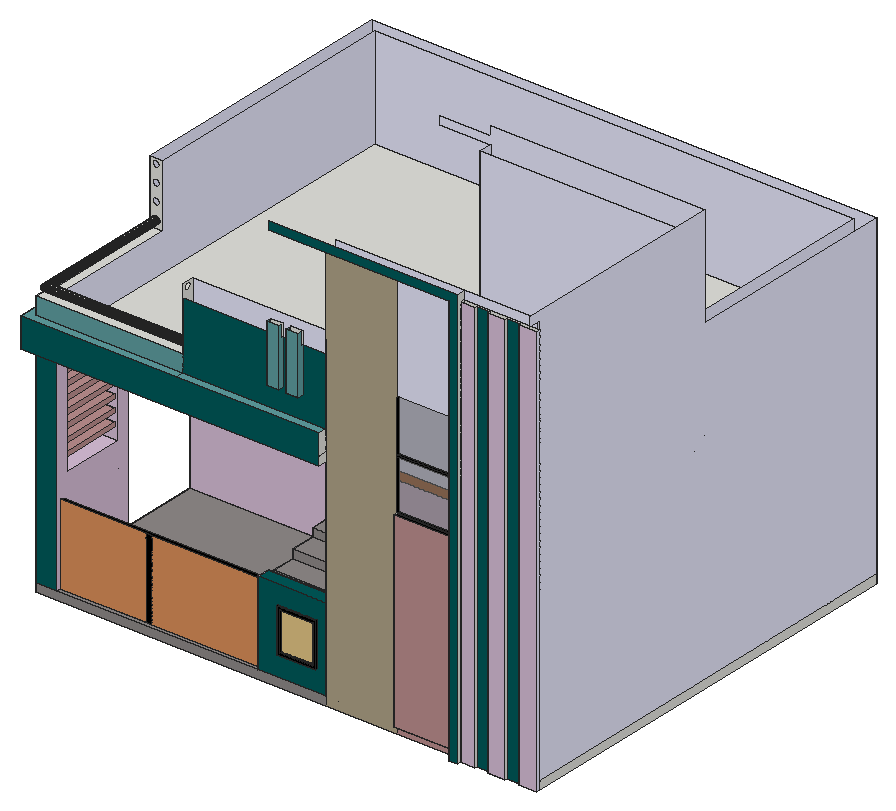
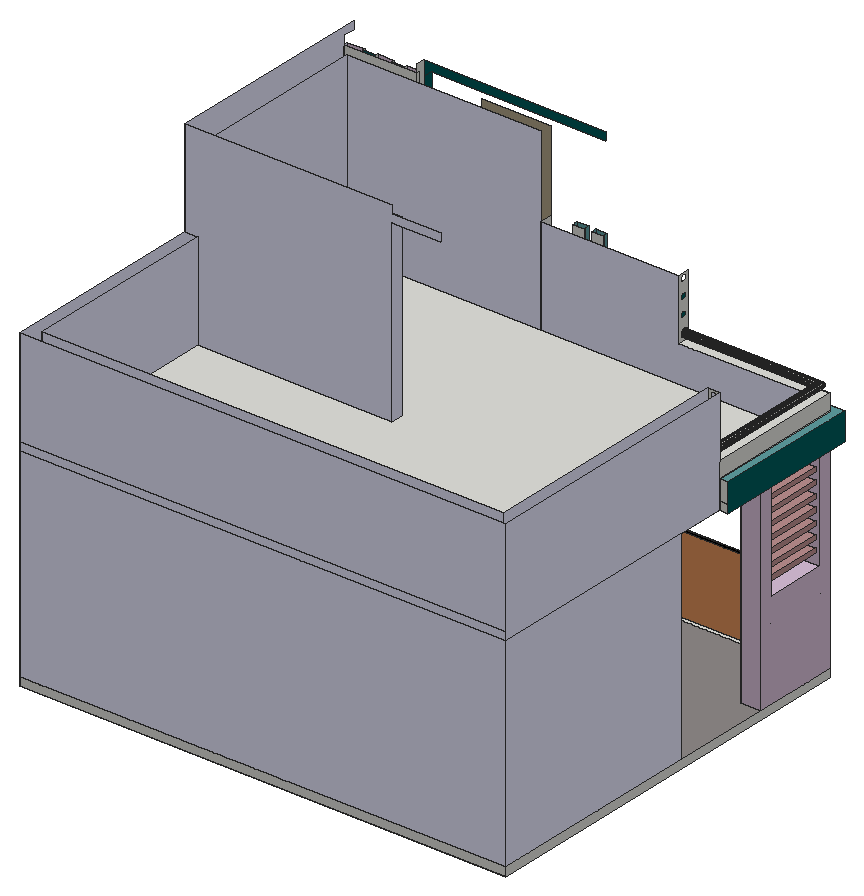
# SketchUp Ruby script. Lengths in inches.
U = 1.inch
M = Sketchup.active_model
def pt(a) = Geom::Point3d.new(a.map { |v| v * U })
def face(e, loops, mat)
  f = e.add_face(loops[0].map { |a| pt(a) })
  loops[1..].each { |l| e.add_face(l.map { |a| pt(a) }).erase! }
  f.material = f.back_material = mat if mat
  f
end
# faces: each face lists its corners as indices into pts; further lists are holes
def faces(e, pts, list, mat = nil) = list.each { |f| face(e, (f[0].is_a?(Array) ? f : [f]).map { |l| l.map { |i| pts[i] } }, mat) }
# xy, xz, yz: faces in a plane at the given z, y or x. An outline is a flat list of corners, or four numbers for a rectangle; further outlines are holes
def ring(l) = l.size == 4 ? [[l[0], l[1]], [l[2], l[1]], [l[2], l[3]], [l[0], l[3]]] : l.each_slice(2).to_a
def flat(e, list, mat, &to3) = list.each { |f| face(e, (f[0].is_a?(Array) ? f : [f]).map { |l| ring(l).map { |u, v| to3.(u, v) } }, mat) }
def xy(e, z, list, mat = nil) = flat(e, list, mat) { |x, y| [x, y, z] }
def xz(e, y, list, mat = nil) = flat(e, list, mat) { |x, z| [x, y, z] }
def yz(e, x, list, mat = nil) = flat(e, list, mat) { |y, z| [x, y, z] }
def lines(e, pts, list) = list.each { |a, b| e.add_line(pt(pts[a]), pt(pts[b])) }
# prism: a flat outline (further loops are holes) pulled along v
def prism(e, loops, v, mat = nil)
  f = face(e, loops, mat); d = Geom::Vector3d.new(v.map { |x| x * U })
  f.pushpull(f.normal.samedirection?(d) ? d.length : -d.length)
end
def box(e, o, s, mat = nil) = prism(e, [[o, [o[0] + s[0], o[1], o[2]], [o[0] + s[0], o[1] + s[1], o[2]], [o[0], o[1] + s[1], o[2]]]], [0, 0, s[2]], mat)
def at(x, y, z, deg = 0) = Geom::Transformation.translation(pt([x, y, z])) * Geom::Transformation.rotation(ORIGIN, Z_AXIS, deg.degrees)
def axes(o, x, y, z) = Geom::Transformation.new([*x, 0, *y, 0, *z, 0, *pt(o).to_a, 1])
def part(name) = M.definitions.add(name)
# library, detail: a bought-in or finely detailed component or shape, given as its bounding box
def library(name, o, s) = part(name).tap { |d| box(d.entities, o, s) }
def detail(e, o, s) = box(e.add_group.entities, o, s)
def put(e, d, t, mat = nil) = e.add_instance(d, t).tap { |i| i.material = mat if mat }
def group(e, t, mat = nil) = e.add_group.tap { |g| g.transformation = t; g.material = mat if mat }.entities
root = M.entities
M.materials.add("[0079_Teal]").color = [0, 91, 91]
M.materials.add("[0080_DarkCyan]").color = [0, 89, 89]
M.materials.add("[0081_CadetBlue]").color = [95, 158, 160]
M.materials.add("[0116_Lavender]").color = [230, 230, 250]
M.materials.add("[0118_Thistle]").color = [216, 191, 216]
M.materials.add("[0119_RosyBrown]").color = [188, 143, 143]
M.materials.add("[0137_Black]").color = [0, 0, 0]
M.materials.add("[Beadboard]").color = [218, 143, 90]
M.materials.add("[Cladding Siding White]").color = [175, 162, 135]
M.materials.add("[Stone Brushed Khaki]").color = [226, 197, 133]
M.materials.add("[Stone Marble]").color = [143, 138, 136]
M.materials.add("[Translucent Glass Gray]").color = [128, 128, 128]
M.materials["[Translucent Glass Gray]"].alpha = 0.5
M.materials.add("[Wood Cherry Original]").color = [152, 86, 42]
xy(root,0,[[12,18,732,618]])
xy(root,0,[[612,6,624,18],[624,12,624,18,732,18,732,12,706.05,12,706.05,15,687.09,15,687.09,12,663.05,12,663.05,15,644.09,15,644.09,12]],"[0119_RosyBrown]")
xy(root,12,[[12,18,42,145.875],[330,18,426,18,426,36,330,36,330,29.83,42,29.83,42,24.27,330,24.27],[42,29.83,330,36],[215.92,187.6875,352.01,294],[12,294,732,618]])
xy(root,12,[[528,12,612,18]],"[0119_RosyBrown]")
xy(root,12,[[42,18,330,24.27],[42,36,714,36,714,294,352.01,294,352.01,187.6875,215.92,187.6875,215.92,294,12,294,12,145.875,42,145.875]],"[Stone Marble]")
xy(root,25,[[215.92,187.6875,352.01,221.8125]],"[Stone Marble]")
xy(root,37,[[215.92,221.8125,352.01,257.5]],"[Stone Marble]")
xy(root,42.64,[[358.44,16,414.07,18]])
xy(root,46.64,[[362.44,16,410.07,18]],"[0137_Black]")
xy(root,49,[[215.92,257.5,352.01,294]],"[Stone Marble]")
xy(root,53.48,[[233.84,294,333.51,297]])
xy(root,101.14,[[362.44,16,410.07,18]],"[0137_Black]")
xy(root,105.14,[[358.44,16,414.07,18]],"[0137_Black]")
xy(root,126.3125,[[42,24.27,330,29.83]],"[0137_Black]")
xy(root,132,[[330,18,426,36]],"[0080_DarkCyan]")
xy(root,139.17,[[105.73,294,141.83,297],[146.88,294,184.78,297]])
xy(root,156,[[12,36,42,127.875]],"[0118_Thistle]")
xy(root,171.26,[[18.41,36,37.6,127.875]])
xy(root,178.13,[[18.41,36,37.6,127.875]],"[0119_RosyBrown]")
xy(root,189.26,[[18.41,36,37.6,127.875]])
xy(root,196.13,[[18.41,36,37.6,127.875]],"[0119_RosyBrown]")
xy(root,207.26,[[18.41,36,37.6,127.875]],"[0119_RosyBrown]")
xy(root,214.13,[[18.41,36,37.6,127.875]],"[0119_RosyBrown]")
xy(root,225.26,[[18.41,36,37.6,127.875]],"[0119_RosyBrown]")
xy(root,232.13,[[18.41,36,37.6,127.875]],"[0119_RosyBrown]")
xy(root,243.26,[[18.41,36,37.6,127.875]],"[0119_RosyBrown]")
xy(root,250.13,[[18.41,36,37.6,127.875]],"[0119_RosyBrown]")
xy(root,250.21,[[105.73,294,141.83,297],[146.88,294,184.78,297],[233.84,294,333.51,297]])
xy(root,261.26,[[18.41,36,37.6,127.875]],"[0119_RosyBrown]")
xy(root,268.13,[[18.41,36,37.6,127.875]],"[0119_RosyBrown]")
xy(root,279.26,[[18.41,36,37.6,127.875]],"[0119_RosyBrown]")
xy(root,282,[[528,12,612,18],[528,18,612,21]],"[0137_Black]")
xy(root,286.13,[[18.41,36,37.6,127.875]],"[0119_RosyBrown]")
xy(root,297.26,[[18.41,36,37.6,127.875]],"[0119_RosyBrown]")
xy(root,304.13,[[18.41,36,37.6,127.875]],"[0119_RosyBrown]")
xy(root,312,[[12,36,42,127.875],[112,50.56,110.49,50.96,109.13,51.74,108.02,52.85,107.24,54.2,106.83,55.72,106.83,57.28,107.23,58.8,108.01,60.15,109.12,61.26,110.47,62.05,111.99,62.45,113.55,62.45,115.07,62.05,116.42,61.27,117.53,60.16,118.32,58.81,118.72,57.3,118.73,55.73,118.32,54.22,117.54,52.86,116.43,51.75,115.08,50.96,113.57,50.56],[229.375,50.56,227.86,50.96,226.5,51.74,225.4,52.85,224.61,54.2,224.2,55.72,224.2,57.28,224.61,58.8,225.39,60.15,226.49,61.26,227.85,62.05,229.36,62.45,230.93,62.45,232.44,62.05,233.8,61.27,234.91,60.16,235.69,58.81,236.1,57.3,236.1,55.73,235.7,54.22,234.92,52.86,233.81,51.75,232.45,50.96,230.94,50.56],[354.75,50.56,353.24,50.96,351.88,51.74,350.77,52.85,349.99,54.2,349.58,55.72,349.58,57.28,349.98,58.8,350.76,60.15,351.87,61.26,353.22,62.05,354.74,62.45,356.3,62.45,357.82,62.05,359.17,61.27,360.28,60.16,361.07,58.81,361.47,57.3,361.48,55.73,361.07,54.22,360.29,52.86,359.18,51.75,357.83,50.96,356.32,50.56],[12,127.875,42,145.875],
  [161.43,136.03,159.91,136.43,158.56,137.21,157.45,138.32,156.66,139.68,156.26,141.1875,156.25,142.75,156.66,144.27,157.44,145.625,158.55,146.73,159.9,147.52,161.41,147.93,162.98,147.93,164.49,147.52,165.85,146.74,166.96,145.64,167.74,144.28,168.15,142.77,168.15,141.2,167.75,139.6875,166.97,138.33,165.86,137.22,164.51,136.4375,162.99,136.03],[300.24,136.03,298.73,136.43,297.37,137.21,296.26,138.32,295.48,139.68,295.07,141.1875,295.07,142.75,295.47,144.27,296.25,145.625,297.36,146.73,298.71,147.52,300.23,147.93,301.79,147.93,303.31,147.52,304.66,146.74,305.77,145.64,306.56,144.28,306.96,142.77,306.97,141.2,306.5625,139.6875,305.78,138.33,304.67,137.22,303.32,136.4375,301.81,136.03]])
xy(root,312,[[[0,6,0,222,12,222,12,18,42,18,42,145.875,12,145.875,12,294,714,294,714,36,426,36,426,6],[229.375,50.56,230.94,50.56,232.45,50.96,233.81,51.75,234.92,52.86,235.7,54.22,236.1,55.73,236.1,57.3,235.69,58.81,234.91,60.16,233.8,61.27,232.44,62.05,230.93,62.45,229.36,62.45,227.85,62.05,226.49,61.26,225.39,60.15,224.61,58.8,224.2,57.28,224.2,55.72,224.61,54.2,225.4,52.85,226.5,51.74,227.86,50.96],[354.75,50.56,356.32,50.56,357.83,50.96,359.18,51.75,360.29,52.86,361.07,54.22,361.48,55.73,361.47,57.3,361.07,58.81,360.28,60.16,359.17,61.27,357.82,62.05,356.3,62.45,354.74,62.45,353.22,62.05,351.87,61.26,350.76,60.15,349.98,58.8,349.58,57.28,349.58,55.72,349.99,54.2,350.77,52.85,351.88,51.74,353.24,50.96],[112,50.56,113.57,50.56,115.08,50.96,116.43,51.75,117.54,52.86,118.32,54.22,118.73,55.73,118.72,57.3,118.32,58.81,117.53,60.16,116.42,61.27,115.07,62.05,113.55,62.45,111.99,62.45,110.47,62.05,109.12,61.26,108.01,60.15,107.23,58.8,106.83,57.28,106.83,55.72,107.24,54.2,108.02,52.85,109.13,51.74,110.49,50.96],[300.24,136.03,301.81,136.03,303.32,136.4375,304.67,137.22,305.78,138.33,306.5625,139.6875,306.97,141.2,306.96,142.77,306.56,144.28,305.77,145.64,304.66,146.74,303.31,147.52,301.79,147.93,300.23,147.93,298.71,147.52,297.36,146.73,296.25,145.625,295.47,144.27,295.07,142.75,295.07,141.1875,295.48,139.68,296.26,138.32,297.37,137.21,298.73,136.43],[161.43,136.03,162.99,136.03,164.51,136.4375,165.86,137.22,166.97,138.33,167.75,139.6875,168.15,141.2,168.15,142.77,167.74,144.28,166.96,145.64,165.85,146.74,164.49,147.52,162.98,147.93,161.41,147.93,159.9,147.52,158.55,146.73,157.44,145.625,156.66,144.27,156.25,142.75,156.26,141.1875,156.66,139.68,157.45,138.32,158.56,137.21,159.91,136.43]]],"[Wood Cherry Original]")
xy(root,324,[[30,36,714,36,714,294,426,294,426,312,714,312,714,600,30,600]])
xy(root,354,[[0,6,222,6,222,18,12,18,12,222,0,222],[222,6,426,18]],"[0081_CadetBlue]")
xy(root,354,[[528,18,612,21]],"[0137_Black]")
xy(root,357,[[528,18,612,21]],"[0137_Black]")
xy(root,378,[[12,18,222,18,222,36,30,36,30,222,12,222]])
xy(root,386.125,[[348.57,10,365.51,18],[376.32,10,393.26,18]],"[0081_CadetBlue]")
xz(root,6,[[612,0,624,0,624,600,354,600,354,588,612,588],[0,312,426,354]],"[0080_DarkCyan]")
xz(root,10,[[348.57,386.125,365.51,468],[376.32,386.125,393.26,468]],"[0081_CadetBlue]")
xz(root,12,[[624,0,644.09,588],[663.05,0,687.09,588],[706.05,0,732,588]],"[0118_Thistle]")
xz(root,12,[[528,12,612,282]],"[0119_RosyBrown]")
xz(root,15,[[644.09,0,663.05,588],[687.09,0,706.05,588]],"[0080_DarkCyan]")
xz(root,16,[[[358.44,42.64,414.07,105.14],[362.44,46.64,410.07,101.14]]],"[0137_Black]")
xz(root,18,[[624,0,732,588],[528,12,612,282],[[358.44,42.64,414.07,105.14],[362.44,46.64,410.07,101.14]],[348.57,386.125,365.51,468],[376.32,386.125,393.26,468]])
xz(root,18,[[12,12,42,312],[[330,12,426,132],[358.44,42.64,414.07,105.14]],[222,354,426,354,426,450,393.26,450,393.26,386.125,376.32,386.125,376.32,450,365.51,450,365.51,386.125,348.57,386.125,348.57,450,222,450]],"[0080_DarkCyan]")
xz(root,18,[[12,354,222,378]],"[0081_CadetBlue]")
xz(root,18,[[528,0,612,12]],"[0119_RosyBrown]")
xz(root,18,[[528,354,612,357]],"[0137_Black]")
xz(root,18,[[426,0,528,588]],"[Cladding Siding White]")
xz(root,18,[[362.44,46.64,410.07,101.14]],"[Stone Brushed Khaki]")
xz(root,18,[[12,0,426,12]],"[Stone Marble]")
xz(root,21,[[528,282,612,354],[528,357,612,429]],"[Translucent Glass Gray]")
xz(root,24.27,[[164.07,12,173.47,126.3125]],"[0137_Black]")
xz(root,24.27,[[42,12,164.07,126.3125],[173.47,12,330,126.3125]],"[Beadboard]")
xz(root,29.83,[[42,12,330,126.3125]],"[Beadboard]")
xz(root,36,[[30,324,30,378,222,378,222,468,426,468,426,324],[426,324,714,588]],"[0116_Lavender]")
xz(root,36,[[330,12,426,132],[426,12,714,312],[[12,156,42,312],[18.41,171.26,37.6,178.13],[18.41,189.26,37.6,196.13],[18.41,207.26,37.6,214.13],[18.41,225.26,37.6,232.13],[18.41,243.26,37.6,250.13],[18.41,261.26,37.6,268.13],[18.41,297.26,37.6,304.13],[18.41,279.26,37.6,286.13]]],"[0118_Thistle]")
xz(root,127.875,[[18.41,171.26,37.6,178.13],[18.41,189.26,37.6,196.13],[18.41,207.26,37.6,214.13],[18.41,225.26,37.6,232.13],[18.41,243.26,37.6,250.13],
  [18.41,261.26,37.6,268.13],[18.41,279.26,37.6,286.13],[18.41,297.26,37.6,304.13]])
xz(root,127.875,[[[12,156,42,312],[18.41,297.26,37.6,304.13],[18.41,279.26,37.6,286.13],[18.41,261.26,37.6,268.13],[18.41,243.26,37.6,250.13],[18.41,225.26,37.6,232.13],[18.41,207.26,37.6,214.13],[18.41,189.26,37.6,196.13],[18.41,171.26,37.6,178.13]]],"[0118_Thistle]")
xz(root,145.875,[[12,12,42,312]],"[0118_Thistle]")
xz(root,187.6875,[[215.92,12,352.01,25]],"[Stone Marble]")
xz(root,221.8125,[[215.92,25,352.01,37]],"[Stone Marble]")
xz(root,222,[[0,312,12,324],[0,324,12,354],[[12,378,30,468],[21.12,455.86,20.59,455.87,20.08,455.94,19.57,456.07,19.07,456.24,18.6,456.47,18.16,456.74,17.74,457.0625,17.36,457.42,17.02,457.82,16.73,458.25,16.48,458.72,16.28,459.2,16.13,459.7,16.04,460.22,16,460.74,16.02,461.26,16.09,461.78,16.21,462.29,16.39,462.78,16.61,463.25,16.89,463.7,17.21,464.11,17.57,464.49,17.97,464.83,18.4,465.125,18.86,465.375,19.34,465.57,19.85,465.72,20.36,465.8125,20.88,465.85,21.41,465.84,21.92,465.77,22.43,465.65,22.93,465.47,23.4,465.24,23.84,464.97,24.26,464.65,24.64,464.29,24.98,463.89,25.27,463.46,25.52,463,25.72,462.51,25.87,462.01,25.96,461.49,26,460.97,25.98,460.45,25.91,459.93,25.79,459.42,25.61,458.93,25.39,458.46,25.11,458.01,24.79,457.6,24.43,457.22,24.03,456.88,23.6,456.58,23.14,456.34,22.66,456.14,22.15,455.99,21.64,455.9],[21.12,431.86,20.59,431.87,20.08,431.94,19.57,432.07,19.07,432.24,18.6,432.47,18.16,432.74,17.74,433.0625,17.36,433.42,17.02,433.82,16.73,434.25,16.48,434.72,16.28,435.2,16.13,435.7,16.04,436.22,16,436.74,16.02,437.26,16.09,437.78,16.21,438.29,16.39,438.78,16.61,439.25,16.89,439.7,17.21,440.11,17.57,440.49,17.97,440.83,18.4,441.125,18.86,441.375,19.34,441.57,19.85,441.72,20.36,441.8125,20.88,441.85,21.41,441.84,21.92,441.77,22.43,441.65,22.93,441.47,23.4,441.24,23.84,440.97,24.26,440.65,24.64,440.29,24.98,439.89,25.27,439.46,25.52,439,25.72,438.51,25.87,438.01,25.96,437.49,26,436.97,25.98,436.45,25.91,435.93,25.79,435.42,25.61,434.93,25.39,434.46,25.11,434.01,24.79,433.6,24.43,433.22,24.03,432.88,23.6,432.58,23.14,432.34,22.66,432.14,22.15,431.99,21.64,431.9],[21.12,407.86,20.59,407.87,20.08,407.94,19.57,408.07,19.07,408.24,18.6,408.47,18.16,408.74,17.74,409.0625,17.36,409.42,17.02,409.82,16.73,410.25,16.48,410.72,16.28,411.2,16.13,411.7,16.04,412.22,16,412.74,16.02,413.26,16.09,413.78,16.21,414.29,16.39,414.78,16.61,415.25,16.89,415.7,17.21,416.11,17.57,416.49,17.97,416.83,18.4,417.125,18.86,417.375,19.34,417.57,19.85,417.72,20.36,417.8125,20.88,417.85,21.41,417.84,21.92,417.77,22.43,417.65,22.93,417.47,23.4,417.24,23.84,416.97,24.26,416.65,24.64,416.29,24.98,415.89,25.27,415.46,25.52,415,25.72,414.51,25.87,414.01,25.96,413.49,26,412.97,25.98,412.45,25.91,411.93,25.79,411.42,25.61,410.93,25.39,410.46,25.11,410.01,24.79,409.6,24.43,409.22,24.03,408.88,23.6,408.58,23.14,408.34,22.66,408.14,22.15,407.99,21.64,407.9],[21.12,383.86,20.59,383.87,20.08,383.94,19.57,384.07,19.07,384.24,18.6,384.47,18.16,384.74,17.74,385.0625,17.36,385.42,17.02,385.82,16.73,386.25,16.48,386.72,16.28,387.2,16.13,387.7,16.04,388.22,16,388.74,16.02,389.26,16.09,389.78,16.21,390.29,16.39,390.78,16.61,391.25,16.89,391.7,17.21,392.11,17.57,392.49,17.97,392.83,18.4,393.125,18.86,393.375,19.34,393.57,19.85,393.72,20.36,393.8125,20.88,393.85,21.41,393.84,21.92,393.77,22.43,393.65,22.93,393.47,23.4,393.24,23.84,392.97,24.26,392.65,24.64,392.29,24.98,391.89,25.27,391.46,25.52,391,25.72,390.51,25.87,390.01,25.96,389.49,26,388.97,25.98,388.45,25.91,387.93,25.79,387.42,25.61,386.93,25.39,386.46,25.11,386.01,24.79,385.6,24.43,385.22,24.03,384.88,23.6,384.58,23.14,384.34,22.66,384.14,22.15,383.99,21.64,383.9]],[21.12,383.86,20.59,383.87,20.08,383.94,19.57,384.07,19.07,384.24,18.6,384.47,18.16,384.74,17.74,385.0625,17.36,385.42,17.02,385.82,16.73,386.25,16.48,386.72,16.28,387.2,16.13,387.7,16.04,388.22,16,388.74,16.02,389.26,16.09,389.78,16.21,390.29,16.39,390.78,16.61,391.25,16.89,391.7,17.21,392.11,17.57,392.49,17.97,392.83,18.4,393.125,18.86,393.375,19.34,393.57,19.85,393.72,20.36,393.8125,20.88,393.85,21.41,393.84,21.92,393.77,22.43,393.65,22.93,393.47,23.4,393.24,23.84,392.97,24.26,392.65,24.64,392.29,24.98,391.89,25.27,391.46,25.52,391,25.72,390.51,25.87,390.01,25.96,389.49,26,388.97,25.98,388.45,25.91,387.93,25.79,387.42,25.61,386.93,25.39,386.46,25.11,386.01,24.79,385.6,24.43,385.22,24.03,384.88,23.6,384.58,23.14,384.34,22.66,384.14,22.15,383.99,21.64,383.9]])
xz(root,257.5,[[215.92,37,352.01,49]],"[Stone Marble]")
xz(root,294,[[215.92,12,352.01,25],[215.92,25,352.01,37],[215.92,37,352.01,49]])
xz(root,294,[[426,324,714,588]],"[0116_Lavender]")
xz(root,294,[[[12,12,215.92,12,215.92,49,229.36,49,229.36,254.6875,337.99,254.6875,337.99,49,352.01,49,352.01,12,714,12,714,312,12,312],[101.26,134.6875,189.26,254.6875]]],"[0118_Thistle]")
xz(root,294,[[[229.36,49,337.99,254.6875],[233.84,53.48,333.51,250.21]],[[101.26,134.6875,189.26,254.6875],[105.73,139.17,184.78,250.21]],[141.83,139.17,146.88,250.21]],"[Wood Cherry Original]")
xz(root,297,[[105.73,139.17,141.83,250.21],[146.88,139.17,184.78,250.21]],"[Translucent Glass Gray]")
xz(root,297,[[233.84,53.48,333.51,250.21]],"[Wood Cherry Original]")
xz(root,312,[[426,324,426,588,354,588,354,600,426,600,426,612,732,612,732,468,714,468,714,324]],"[0116_Lavender]")
xz(root,600,[[30,324,714,468]],"[0116_Lavender]")
xz(root,618,[[12,0,732,12]])
xz(root,618,[[12,12,732,312],[12,312,732,324],[12,324,732,468]],"[0116_Lavender]")
yz(root,0,[[6,312,222,354]],"[0079_Teal]")
yz(root,12,[[18,0,618,12],[18,312,222,354],[18,354,222,378]])
yz(root,12,[[294,12,618,312],[222,312,618,468]],"[0116_Lavender]")
yz(root,12,[[18,12,18,312,36,312,36,156,127.875,156,127.875,312,145.875,312,145.875,12]],"[0118_Thistle]")
yz(root,18.41,[[36,171.26,127.875,178.13],[36,189.26,127.875,196.13],[36,207.26,127.875,214.13],[36,225.26,127.875,232.13],[36,243.26,127.875,250.13],
  [36,261.26,127.875,268.13],[36,279.26,127.875,286.13],[36,297.26,127.875,304.13]],"[0119_RosyBrown]")
yz(root,30,[[36,324,600,324,600,468,222,468,222,378,36,378]],"[0116_Lavender]")
yz(root,37.6,[[36,171.26,127.875,178.13],[36,189.26,127.875,196.13],[36,207.26,127.875,214.13],[36,225.26,127.875,232.13],[36,243.26,127.875,250.13],
  [36,261.26,127.875,268.13],[36,279.26,127.875,286.13],[36,297.26,127.875,304.13]],"[0119_RosyBrown]")
yz(root,42,[[18,12,24.27,12,24.27,126.3125,29.83,126.3125,29.83,12,145.875,12,145.875,312,127.875,312,127.875,156,36,156,36,312,18,312]],"[0118_Thistle]")
yz(root,105.73,[[294,139.17,297,250.21]])
yz(root,141.83,[[294,139.17,297,250.21]])
yz(root,146.88,[[294,139.17,297,250.21]])
yz(root,184.78,[[294,139.17,297,250.21]])
yz(root,215.92,[[187.6875,12,187.6875,25,221.8125,25,221.8125,37,257.5,37,257.5,49,294,49,294,12]],"[Stone Marble]")
yz(root,222,[[[18,378,36,468],[26.48,455.86,27.52,455.86,28.04,455.95,28.55,456.08,29.03,456.27,29.5,456.51,29.9375,456.79,30.35,457.12,30.72,457.49,31.05,457.9,31.33,458.34,31.57,458.8,31.76,459.29,31.79,459.42,31.89,459.8,31.91,459.91,31.92,460,31.97,460.3125,31.98,460.4,31.99,460.61,32,460.84,32,460.9,31.98,461.22,31.97,461.36,31.97,461.4,31.9,461.82,31.89,461.875,31.89,461.89,31.76,462.38,31.57,462.87,31.33,463.34,31.05,463.77,30.72,464.18,30.35,464.55,29.9375,464.88,29.5,465.17,29.03,465.4,28.55,465.59,28.04,465.73,27.52,465.81,27,465.84,26.48,465.81,25.96,465.73,25.45,465.59,24.97,465.4,24.5,465.17,24.0625,464.88,23.65,464.55,23.28,464.18,22.95,463.77,22.67,463.34,22.43,462.87,22.24,462.38,22.11,461.88,22.11,461.87,22.04,461.45,22.03,461.36,22.03,461.33,22.01,461.02,22,460.84,22,460.78,22.01,460.58,22.03,460.3125,22.04,460.24,22.05,460.14,22.11,459.8,22.13,459.7,22.24,459.29,22.43,458.8,22.67,458.34,22.95,457.9,23.28,457.49,23.65,457.12,24.0625,456.79,24.5,456.51,24.97,456.27,25.45,456.08,25.96,455.95],[26.48,431.86,27.52,431.86,28.04,431.95,28.55,432.08,29.03,432.27,29.5,432.51,29.9375,432.79,30.35,433.12,30.72,433.49,31.05,433.9,31.33,434.34,31.57,434.8,31.76,435.29,31.79,435.42,31.89,435.8,31.91,435.91,31.92,436,31.97,436.3125,31.98,436.4,31.99,436.61,32,436.84,32,436.9,31.98,437.22,31.97,437.36,31.97,437.4,31.9,437.82,31.89,437.875,31.89,437.89,31.76,438.38,31.57,438.87,31.33,439.34,31.05,439.77,30.72,440.18,30.35,440.55,29.9375,440.88,29.5,441.17,29.03,441.4,28.55,441.59,28.04,441.73,27.52,441.81,27,441.84,26.48,441.81,25.96,441.73,25.45,441.59,24.97,441.4,24.5,441.17,24.0625,440.88,23.65,440.55,23.28,440.18,22.95,439.77,22.67,439.34,22.43,438.87,22.24,438.38,22.11,437.88,22.11,437.87,22.04,437.45,22.03,437.36,22.03,437.33,22.01,437.02,22,436.84,22,436.78,22.01,436.58,22.03,436.3125,22.04,436.24,22.05,436.14,22.11,435.8,22.13,435.7,22.24,435.29,22.43,434.8,22.67,434.34,22.95,433.9,23.28,433.49,23.65,433.12,24.0625,432.79,24.5,432.51,24.97,432.27,25.45,432.08,25.96,431.95],[26.48,407.86,27.52,407.86,28.04,407.95,28.55,408.08,29.03,408.27,29.5,408.51,29.9375,408.79,30.35,409.12,30.72,409.49,31.05,409.9,31.33,410.34,31.57,410.8,31.76,411.29,31.79,411.42,31.89,411.8,31.91,411.91,31.92,412,31.97,412.3125,31.98,412.4,31.99,412.61,32,412.84,32,412.9,31.98,413.22,31.97,413.36,31.97,413.4,31.9,413.82,31.89,413.875,31.89,413.89,31.76,414.38,31.57,414.87,31.33,415.34,31.05,415.77,30.72,416.18,30.35,416.55,29.9375,416.88,29.5,417.17,29.03,417.4,28.55,417.59,28.04,417.73,27.52,417.81,27,417.84,26.48,417.81,25.96,417.73,25.45,417.59,24.97,417.4,24.5,417.17,24.0625,416.88,23.65,416.55,23.28,416.18,22.95,415.77,22.67,415.34,22.43,414.87,22.24,414.38,22.11,413.88,22.11,413.87,22.04,413.45,22.03,413.36,22.03,413.33,22.01,413.02,22,412.84,22,412.78,22.01,412.58,22.03,412.3125,22.04,412.24,22.05,412.14,22.11,411.8,22.13,411.7,22.24,411.29,22.43,410.8,22.67,410.34,22.95,409.9,23.28,409.49,23.65,409.12,24.0625,408.79,24.5,408.51,24.97,408.27,25.45,408.08,25.96,407.95],[26.48,383.86,27.52,383.86,28.04,383.95,28.55,384.08,29.03,384.27,29.5,384.51,29.9375,384.79,30.35,385.12,30.72,385.49,31.05,385.9,31.33,386.34,31.57,386.8,31.76,387.29,31.79,387.42,31.89,387.8,31.91,387.91,31.92,388,31.97,388.3125,31.98,388.4,31.99,388.61,32,388.84,32,388.9,31.98,389.22,31.97,389.36,31.97,389.4,31.9,389.82,31.89,389.875,31.89,389.89,31.76,390.38,31.57,390.87,31.33,391.34,31.05,391.77,30.72,392.18,30.35,392.55,29.9375,392.88,29.5,393.17,29.03,393.4,28.55,393.59,28.04,393.73,27.52,393.81,27,393.84,26.48,393.81,25.96,393.73,25.45,393.59,24.97,393.4,24.5,393.17,24.0625,392.88,23.65,392.55,23.28,392.18,22.95,391.77,22.67,391.34,22.43,390.87,22.24,390.38,22.11,389.88,22.11,389.87,22.04,389.45,22.03,389.36,22.03,389.33,22.01,389.02,22,388.84,22,388.78,22.01,388.58,22.03,388.3125,22.04,388.24,22.05,388.14,22.11,387.8,22.13,387.7,22.24,387.29,22.43,386.8,22.67,386.34,22.95,385.9,23.28,385.49,23.65,385.12,24.0625,384.79,24.5,384.51,24.97,384.27,25.45,384.08,25.96,383.95]],[26.48,383.86,25.96,383.95,25.45,384.08,24.97,384.27,24.5,384.51,24.0625,384.79,23.65,385.12,23.28,385.49,22.95,385.9,22.67,386.34,22.43,386.8,22.24,387.29,22.13,387.7,22.11,387.8,22.05,388.14,22.13,387.7,22.28,387.2,22.48,386.72,22.73,386.25,23.02,385.82,23.36,385.42,23.74,385.0625,24.16,384.74,24.6,384.47,25.07,384.24,25.57,384.07,26.08,383.94,26.59,383.87,27.08,383.86],[27.14,383.86,27.64,383.9,28.15,383.99,28.66,384.14,29.14,384.34,29.6,384.58,30.03,384.88,30.43,385.22,30.79,385.6,31.11,386.01,31.39,386.46,31.61,386.93,31.79,387.42,31.91,387.91,31.89,387.8,31.79,387.42,31.76,387.29,31.57,386.8,31.33,386.34,31.05,385.9,30.72,385.49,30.35,385.12,29.9375,384.79,29.5,384.51,29.03,384.27,28.55,384.08,28.04,383.95,27.52,383.86],[31.92,388,31.98,388.4,31.97,388.3125],[22.04,388.24,22.03,388.3125,22.01,388.58],
  [31.99,388.61,32,388.9,32,388.84],[22,388.78,22,388.84,22.01,389.02],[31.98,389.22,31.97,389.4,31.97,389.36],[22.03,389.33,22.03,389.36,22.04,389.45],[31.9,389.82,31.89,389.89,31.89,389.875]])
yz(root,233.84,[[294,53.48,297,250.21]])
yz(root,330,[[18,12,18,132,36,132,36,12,29.83,12,29.83,126.3125,24.27,126.3125,24.27,12]],"[0118_Thistle]")
yz(root,333.51,[[294,53.48,297,250.21]])
yz(root,348.57,[[10,386.125,10,468,14,468,14,450,18,450,18,386.125]],"[0081_CadetBlue]")
yz(root,352.01,[[187.6875,12,294,12,294,49,257.5,49,257.5,37,221.8125,37,221.8125,25,187.6875,25]],"[Stone Marble]")
yz(root,358.44,[[16,42.64,18,105.14]],"[0137_Black]")
yz(root,362.44,[[16,46.64,18,101.14]],"[0137_Black]")
yz(root,365.51,[[10,386.125,18,386.125,18,450,14,450,14,468,10,468]],"[0081_CadetBlue]")
yz(root,376.32,[[10,386.125,10,468,14,468,14,450,18,450,18,386.125]],"[0081_CadetBlue]")
yz(root,393.26,[[10,386.125,18,386.125,18,450,14,450,14,468,10,468]],"[0081_CadetBlue]")
yz(root,410.07,[[16,46.64,18,101.14]],"[0137_Black]")
yz(root,414.07,[[16,42.64,18,105.14]],"[0137_Black]")
yz(root,426,[[18,12,36,132],[6,312,18,324],[6,324,18,354],[18,324,36,468]])
yz(root,426,[[294,324,312,588]],"[0116_Lavender]")
yz(root,426,[[18,132,36,312]],"[0118_Thistle]")
yz(root,528,[[12,12,18,282]])
yz(root,528,[[18,282,21,354],[18,357,21,429]],"[0137_Black]")
yz(root,612,[[12,12,18,282]])
yz(root,612,[[6,0,6,588,18,588,18,504,21,504,21,432,18,432,18,429,21,429,21,357,18,357,18,354,21,354,21,282,12,282,12,12,18,12,18,0]],"[0080_DarkCyan]")
yz(root,624,[[6,0,12,0,12,588,18,588,18,600,6,600],[12,0,18,588]])
yz(root,644.09,[[12,0,15,588]])
yz(root,663.05,[[12,0,15,588]])
yz(root,687.09,[[12,0,15,588]])
yz(root,706.05,[[12,0,15,588]])
yz(root,714,[[36,324,294,588],[312,324,600,468]],"[0116_Lavender]")
yz(root,714,[[36,12,294,312]],"[0118_Thistle]")
yz(root,732,[[18,0,618,12]])
yz(root,732,[[12,0,18,588],[18,12,618,12,618,468,312,468,312,612,0,612,0,600,18,600]],"[0116_Lavender]")
p = [[19.57,222,384.07],[20.08,222,383.94],[20.08,26.08,383.94],[19.57,25.57,384.07],[222,26.08,383.94],[222,25.57,384.07],
  [20.59,222,383.87],[20.59,26.59,383.87],[222,26.59,383.87],[21.12,222,383.86],[21.12,27.12,383.86],[222,27.12,383.86],
  [222,27.08,383.86],[21.64,222,383.9],[21.64,27.64,383.9],[222,27.64,383.9],[222,27.14,383.86],[22.15,222,383.99],
  [22.15,28.15,383.99],[222,28.15,383.99],[22.66,222,384.14],[22.66,28.66,384.14],[222,28.66,384.14],[19.07,222,384.24],
  [19.07,25.07,384.24],[222,25.07,384.24],[23.14,222,384.34],[23.14,29.14,384.34],[222,29.14,384.34],[18.6,222,384.47],
  [18.6,24.6,384.47],[222,24.6,384.47],[23.6,222,384.58],[23.6,29.6,384.58],[222,29.6,384.58],[18.16,222,384.74],
  [18.16,24.16,384.74],[222,24.16,384.74],[24.03,222,384.88],[24.03,30.03,384.88],[222,30.03,384.88],[17.74,222,385.0625],
  [17.74,23.74,385.0625],[222,23.74,385.0625],[24.43,222,385.22],[24.43,30.43,385.22],[222,30.43,385.22],[17.36,222,385.42],
  [17.36,23.36,385.42],[222,23.36,385.42],[24.79,222,385.6],[24.79,30.79,385.6],[222,30.79,385.6],[17.02,222,385.82],
  [17.02,23.02,385.82],[222,23.02,385.82],[25.11,222,386.01],[25.11,31.11,386.01],[222,31.11,386.01],[16.73,222,386.25],
  [16.73,22.73,386.25],[222,22.73,386.25],[25.39,222,386.46],[25.39,31.39,386.46],[222,31.39,386.46],[16.48,222,386.72],
  [16.48,22.48,386.72],[222,22.48,386.72],[25.61,222,386.93],[25.61,31.61,386.93],[222,31.61,386.93],[16.28,222,387.2],
  [16.28,22.28,387.2],[222,22.28,387.2],[25.79,222,387.42],[25.79,31.79,387.42],[222,31.79,387.42],[16.13,222,387.7],
  [16.13,22.13,387.7],[222,22.13,387.7],[25.91,222,387.93],[25.91,31.91,387.93],[222,31.91,387.93],[222,31.91,387.91],
  [16.04,222,388.22],[16.04,22.04,388.22],[222,22.05,388.14],[222,22.04,388.22],[25.98,222,388.45],[25.98,31.98,388.45],
  [222,31.98,388.45],[222,31.98,388.4],[222,31.92,388],[16,222,388.74],[16,22,388.74],[222,22.04,388.24],
  [222,22.01,388.58],[222,22,388.74],[26,222,388.97],[26,32,388.97],[222,32,388.97],[222,32,388.9],
  [222,31.99,388.61],[16.02,222,389.26],[16.02,22.02,389.26],[222,22,388.78],[222,22.01,389.02],[222,22.02,389.26],
  [25.96,222,389.49],[25.96,31.96,389.49],[222,31.96,389.49],[222,31.97,389.4],[222,31.98,389.22],[16.09,222,389.78],
  [16.09,22.09,389.78],[222,22.03,389.33],[222,22.04,389.45],[222,22.09,389.78],[25.87,222,390.01],[25.87,31.87,390.01],
  [222,31.87,390.01],[222,31.89,389.89],[222,31.9,389.82],[16.21,222,390.29],[16.21,22.21,390.29],[222,22.11,389.87],
  [222,22.11,389.875],[222,22.11,389.88],[222,22.21,390.29],[25.72,222,390.51],[25.72,31.72,390.51],[222,31.72,390.51],
  [222,31.76,390.38],[16.39,222,390.78],[16.39,22.39,390.78],[222,22.39,390.78],[25.52,222,391],[25.52,31.52,391],
  [222,31.52,391],[16.61,222,391.25],[16.61,22.61,391.25],[222,22.61,391.25],[25.27,222,391.46],[25.27,31.27,391.46],
  [222,31.27,391.46],[16.89,222,391.7],[16.89,22.89,391.7],[222,22.89,391.7],[24.98,222,391.89],[24.98,30.98,391.89],
  [222,30.98,391.89],[17.21,222,392.11],[17.21,23.21,392.11],[222,23.21,392.11],[24.64,222,392.29],[24.64,30.64,392.29],
  [222,30.64,392.29],[17.57,222,392.49],[17.57,23.57,392.49],[222,23.57,392.49],[24.26,222,392.65],[24.26,30.26,392.65],
  [222,30.26,392.65],[17.97,222,392.83],[17.97,23.97,392.83],[222,23.97,392.83],[23.84,222,392.97],[23.84,29.84,392.97],
  [222,29.84,392.97],[18.4,222,393.125],[18.4,24.4,393.125],[222,24.4,393.125],[23.4,222,393.24],[23.4,29.4,393.24],
  [222,29.4,393.24],[18.86,222,393.375],[18.86,24.86,393.375],[222,24.86,393.375],[22.93,222,393.47],[22.93,28.93,393.47],
  [222,28.93,393.47],[19.34,222,393.57],[19.34,25.34,393.57],[222,25.34,393.57],[22.43,222,393.65],[22.43,28.43,393.65],
  [222,28.43,393.65],[19.85,222,393.72],[19.85,25.85,393.72],[222,25.85,393.72],[21.92,222,393.77],[21.92,27.92,393.77],
  [222,27.92,393.77],[20.36,222,393.8125],[20.36,26.36,393.8125],[222,26.36,393.8125],[20.88,222,393.85],[20.88,26.88,393.85],
  [222,26.88,393.85],[21.41,222,393.84],[21.41,27.41,393.84],[222,27.41,393.84],[732,294,312],[714,294,312],
  [444,18,12],[444,36,12],[714,312,324],[732,312,324],[12,127.875,120],[42,127.875,120],
  [42,36,120],[12,36,120],[21,222,388.86],[21,27,388.86],[222,27,388.86]]
faces(root,p,[[0,1,2,3],[3,2,4,5],[1,6,7,2],[2,7,8,4],[6,9,10,7],[7,10,11,12,8],[9,13,14,10],[10,14,15,16,11],
  [13,17,18,14],[14,18,19,15],[17,20,21,18],[18,21,22,19],[23,0,3,24],[24,3,5,25],[20,26,27,21],[21,27,28,22],
  [29,23,24,30],[30,24,25,31],[26,32,33,27],[27,33,34,28],[35,29,30,36],[36,30,31,37],[32,38,39,33],[33,39,40,34],
  [41,35,36,42],[42,36,37,43],[38,44,45,39],[39,45,46,40],[47,41,42,48],[48,42,43,49],[44,50,51,45],[45,51,52,46],
  [53,47,48,54],[54,48,49,55],[50,56,57,51],[51,57,58,52],[59,53,54,60],[60,54,55,61],[56,62,63,57],[57,63,64,58],
  [65,59,60,66],[66,60,61,67],[62,68,69,63],[63,69,70,64],[71,65,66,72],[72,66,67,73],[68,74,75,69],[69,75,76,70],
  [77,71,72,78],[78,72,73,79],[74,80,81,75],[75,81,82,83,76],[84,77,78,85],[85,78,79,86,87],[80,88,89,81],[81,89,90,91,92,82],
  [93,84,85,94],[94,85,87,95,96,97],[88,98,99,89],[89,99,100,101,102,90],[103,93,94,104],[104,94,97,105,106,107],[98,108,109,99],[99,109,110,111,112,100],
  [113,103,104,114],[114,104,107,115,116,117],[108,118,119,109],[109,119,120,121,122,110],[123,113,114,124],[124,114,117,125,126,127,128],[118,129,130,119],[119,130,131,132,120],
  [133,123,124,134],[134,124,128,135],[129,136,137,130],[130,137,138,131],[139,133,134,140],[140,134,135,141],[136,142,143,137],[137,143,144,138],
  [145,139,140,146],[146,140,141,147],[142,148,149,143],[143,149,150,144],[151,145,146,152],[152,146,147,153],[148,154,155,149],[149,155,156,150],
  [157,151,152,158],[158,152,153,159],[154,160,161,155],[155,161,162,156],[163,157,158,164],[164,158,159,165],[160,166,167,161],[161,167,168,162],
  [169,163,164,170],[170,164,165,171],[166,172,173,167],[167,173,174,168],[175,169,170,176],[176,170,171,177],[172,178,179,173],[173,179,180,174],
  [181,175,176,182],[182,176,177,183],[178,184,185,179],[179,185,186,180],[187,181,182,188],[188,182,183,189],[184,190,191,185],[185,191,192,186],
  [193,187,188,194],[194,188,189,195],[196,193,194,197],[197,194,195,198],[199,196,197,200],[200,197,198,201],[190,199,200,191],[191,200,201,192]])
lines(root,p,[[202,203],[204,205],[206,207],[208,209],[210,211],[212,213],[213,214]])
